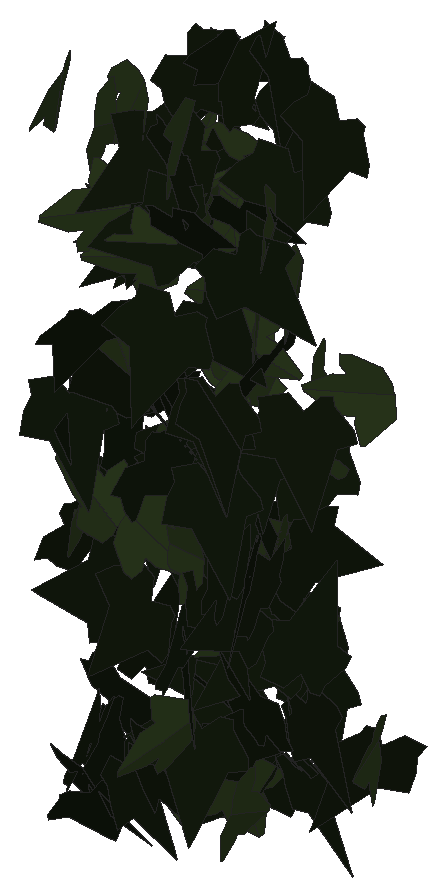
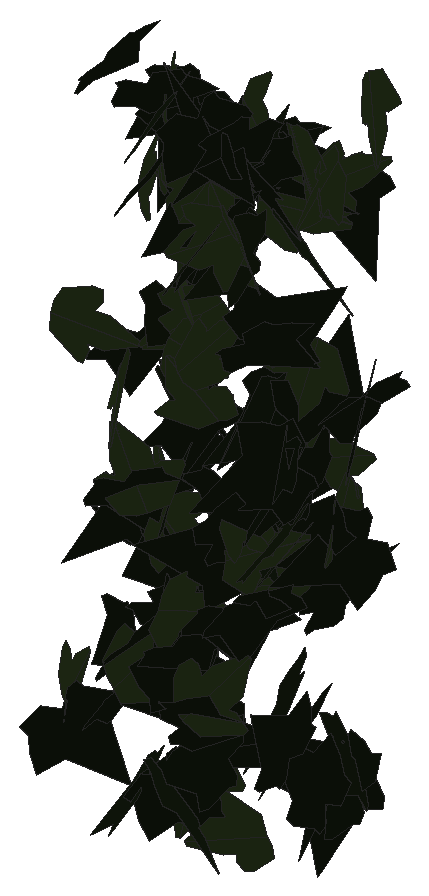
# SketchUp Ruby script. Lengths in inches.
U = 1.inch
M = Sketchup.active_model
def pt(a) = Geom::Point3d.new(a.map { |v| v * U })
def face(e, loops, mat)
  f = e.add_face(loops[0].map { |a| pt(a) })
  loops[1..].each { |l| e.add_face(l.map { |a| pt(a) }).erase! }
  f.material = f.back_material = mat if mat
  f
end
# faces: each face lists its corners as indices into pts; further lists are holes
def faces(e, pts, list, mat = nil) = list.each { |f| face(e, (f[0].is_a?(Array) ? f : [f]).map { |l| l.map { |i| pts[i] } }, mat) }
# xy, xz, yz: faces in a plane at the given z, y or x. An outline is a flat list of corners, or four numbers for a rectangle; further outlines are holes
def ring(l) = l.size == 4 ? [[l[0], l[1]], [l[2], l[1]], [l[2], l[3]], [l[0], l[3]]] : l.each_slice(2).to_a
def flat(e, list, mat, &to3) = list.each { |f| face(e, (f[0].is_a?(Array) ? f : [f]).map { |l| ring(l).map { |u, v| to3.(u, v) } }, mat) }
def xy(e, z, list, mat = nil) = flat(e, list, mat) { |x, y| [x, y, z] }
def xz(e, y, list, mat = nil) = flat(e, list, mat) { |x, z| [x, y, z] }
def yz(e, x, list, mat = nil) = flat(e, list, mat) { |y, z| [x, y, z] }
def lines(e, pts, list) = list.each { |a, b| e.add_line(pt(pts[a]), pt(pts[b])) }
# prism: a flat outline (further loops are holes) pulled along v
def prism(e, loops, v, mat = nil)
  f = face(e, loops, mat); d = Geom::Vector3d.new(v.map { |x| x * U })
  f.pushpull(f.normal.samedirection?(d) ? d.length : -d.length)
end
def box(e, o, s, mat = nil) = prism(e, [[o, [o[0] + s[0], o[1], o[2]], [o[0] + s[0], o[1] + s[1], o[2]], [o[0], o[1] + s[1], o[2]]]], [0, 0, s[2]], mat)
def at(x, y, z, deg = 0) = Geom::Transformation.translation(pt([x, y, z])) * Geom::Transformation.rotation(ORIGIN, Z_AXIS, deg.degrees)
def axes(o, x, y, z) = Geom::Transformation.new([*x, 0, *y, 0, *z, 0, *pt(o).to_a, 1])
def part(name) = M.definitions.add(name)
# library, detail: a bought-in or finely detailed component or shape, given as its bounding box
def library(name, o, s) = part(name).tap { |d| box(d.entities, o, s) }
def detail(e, o, s) = box(e.add_group.entities, o, s)
def put(e, d, t, mat = nil) = e.add_instance(d, t).tap { |i| i.material = mat if mat }
def group(e, t, mat = nil) = e.add_group.tap { |g| g.transformation = t; g.material = mat if mat }.entities
root = M.entities
M.materials.add("efeu1").color = [18, 25, 13]
M.materials.add("efeu2").color = [43, 57, 29]
c1 = part("ivyleaf_9")
p = [[1.54,2.16,1.25],[1.36,2.04,1.19],[-0.21,0.99,0.68],[-0.71,1.11,0.82],[-0.85,0.86,0.67],[-0.8,0.17,0.21],
  [-0.9,-0.01,0.1],[-0.67,-0.16,-0.02],[-0.08,-0.08,-0.05],[-0.03,-0.6,-0.4],[0.65,-0.88,-0.66],[0.83,-0.6,-0.49],
  [1.29,-0.42,-0.43],[1.8125,-0.07,-0.26],[1.21,0.44,0.15]]
faces(c1.entities,p,[[0,1,2,3,4,5,6,7,8,9,10,11,12,13,14]],"efeu1")
c2 = part("ivyleaf_10")
p = [[0,0.5,-0.03],[-0.0625,2.02,-0.43],[-0.19,2.01,-0.46],[-0.54,1.05,-0.29],[-0.52,0.625,-0.18],[-0.83,0.76,-0.28],
  [-1.16,0.64,-0.33],[-1.15,0.33,-0.24],[-0.77,-0.39,0.02],[-0.3,-0.51,0.16],[0.04,-0.48,0.23],[-0.02,2.01,-0.4375],
  [-0.06,2.01,-0.43],[0.04,-0.49,0.23],[0.67,-0.49,0.14],[1.38,0.36,-0.2],[1.375,0.51,-0.24],[0.81,0.65,-0.19],
  [0.62,0.59,-0.15],[0.6,1.09,-0.28],[0.5,1.23,-0.31]]
faces(c2.entities,p,[[0,1,2,3,4,5,6,7,8,9,10],[11,12,0,13,14,15,16,17,18,19,20]],"efeu2")
put(root,c1,axes([37.8,221.21,223.68],[0.09366,-0.09752,0.48137],[0.35058,-0.32993,-0.13506],[0.34398,0.36281,0.00657]))
put(root,c1,axes([38.375,219.91,223.58],[0.02364,0.24467,0.43541],[-0.069,0.43331,-0.23974],[-0.49465,-0.04875,0.05425]))
put(root,c2,axes([38.27,219.55,233.58],[0.1026,-0.46256,-0.15972],[-0.0382,0.15512,-0.47379],[0.48787,0.10943,-0.00351]))
put(root,c1,axes([38.21,221.43,224.3],[-0.06862,-0.15046,0.47186],[0.23997,0.40661,0.16456],[-0.43325,0.24905,0.01641]))
put(root,c1,axes([38.37,220.29,223.71],[0.09712,-0.08424,-0.48319],[-0.36952,0.31133,-0.12855],[0.32252,0.38207,-0.00178]))
put(root,c2,axes([38.31,220.36,232.64],[0.01185,-0.19518,-0.46018],[0.03052,0.45973,-0.19421],[0.49893,-0.02348,0.02281]))
put(root,c1,axes([38.17,219.9,226.92],[-0.0158,0.1862,-0.46376],[-0.03618,0.46235,0.18687],[0.49844,0.03946,-0.00114]))
put(root,c1,axes([38.4,222.04,230.77],[-0.32041,-0.35269,0.15149],[-0.10331,-0.11081,-0.4765],[0.36968,-0.33665,-0.00187]))
put(root,c1,axes([38.34,219.93,228.12],[-0.06556,0.01767,0.49537],[-0.03154,-0.49882,0.01362],[0.49468,-0.02946,0.06652]))
put(root,c1,axes([38.74,221.24,230.4],[0.08388,-0.01017,0.49281],[-0.4844,0.09082,0.08432],[-0.09123,-0.49158,0.00539]))
put(root,c2,axes([38.51,219.78,227.43],[0.06408,-0.33011,-0.37003],[0.00126,0.37322,-0.33273],[0.49588,0.04171,0.04866]))
put(root,c1,axes([38.6,220.32,225.93],[-0.105,-0.08425,0.48154],[-0.2914,-0.38467,-0.13084],[0.39251,-0.30812,0.03168]))
put(root,c1,axes([38.35,219.69,228.93],[0.02029,-0.48656,-0.11337],[0.01966,0.11415,-0.4864],[0.4992,0.01528,0.02376]))
put(root,c1,axes([38.58,220.46,227.85],[-0.04029,-0.15588,0.47337],[0.16236,0.4449,0.16033],[-0.47119,0.16663,0.01477]))
put(root,c1,axes([38.15,220.0625,223.17],[0.33116,-0.23651,0.29051],[0.24227,-0.16053,-0.40686],[0.28572,0.41024,0.00828]))
put(root,c2,axes([38.67,220.6,233.11],[0.38557,-0.25448,-0.19124],[-0.13642,0.13931,-0.46041],[0.28761,0.40723,0.038]))
put(root,c1,axes([38.66,219.77,223.23],[0.22546,0.44087,-0.06926],[-0.04183,-0.05638,-0.49505],[-0.44432,0.22903,0.01146]))
put(root,c1,axes([38.59,220.16,228.7],[0.37372,0.11242,0.31256],[-0.30078,-0.08507,0.39025],[0.14092,-0.47971,0.00404]))
put(root,c1,axes([38.6,221.04,228.71],[0.42532,-0.0676,-0.25404],[-0.25288,0.02676,-0.43051],[0.0718,0.49469,-0.01143]))
put(root,c1,axes([38.58,221.75,226.57],[-0.08422,-0.46567,-0.16143],[0.01454,0.16135,-0.47303],[0.49264,-0.08437,-0.01363]))
put(root,c1,axes([38.45,221.09,228.47],[0.40359,0.16044,0.24773],[0.21602,0.1254,-0.43314],[-0.20112,0.45666,0.0319]))
put(root,c1,axes([38.56,221.07,227.08],[0.0755,-0.45992,0.18102],[0.04637,-0.17572,-0.4658],[0.49209,0.08712,0.01612]))
put(root,c1,axes([38.6,221.46,227.22],[-0.03424,-0.39071,0.31011],[0.09378,-0.31034,-0.38065],[0.48993,0.0321,0.09453]))
put(root,c2,axes([39.12,219.48,227.64],[0.24319,0.08323,0.42887],[-0.43098,-0.03466,0.25111],[0.07152,-0.4918,0.05488]))
put(root,c2,axes([38.82,220.2,229.63],[-0.49191,-0.05886,-0.06754],[0.06744,0.00491,-0.49541],[0.05898,-0.4965,0.00311]))
put(root,c2,axes([38.98,221.47,227.13],[0.02043,0.03241,-0.49853],[-0.29026,-0.40532,-0.03824],[-0.40661,0.29097,0.00225]))
put(root,c1,axes([39.04,221.88,227.48],[-0.14516,-0.05957,0.47474],[-0.37338,-0.29612,-0.15132],[0.29919,-0.39845,0.04148]))
put(root,c1,axes([38.6,220.49,226.93],[-0.15026,-0.00193,0.47688],[0.47683,0.00755,0.15027],[-0.00778,0.49994,-0.00043]))
put(root,c1,axes([38.77,222,226.58],[-0.17085,-0.45556,-0.1152],[0.0422,0.10721,-0.48654],[0.468,-0.17598,0.00181]))
put(root,c2,axes([38.89,221.61,227.87],[-0.00604,-0.39503,0.30645],[0.05429,-0.30518,-0.39232],[0.49701,0.02853,0.04658]))
put(root,c2,axes([39,219.68,231.93],[-0.01634,0.10126,0.48937],[-0.08212,-0.48352,0.09731],[0.49294,-0.07719,0.03243]))
put(root,c2,axes([38.76,221.61,231.53],[0.41683,-0.2476,-0.12224],[0.11745,-0.04133,0.48425],[-0.24991,-0.43242,0.02371]))
put(root,c1,axes([39.23,220.17,231.45],[-0.4315,0.2526,0.00107],[-0.0024,-0.00198,-0.49999],[-0.25259,-0.4315,0.00292]))
put(root,c1,axes([38.86,221.43,231.72],[0.4296,-0.25429,0.02784],[0.02809,-0.00719,-0.49916],[0.25427,0.43044,0.0081]))
put(root,c1,axes([39.33,220.45,232.51],[-0.27676,-0.29301,0.29589],[-0.20834,-0.2102,-0.40301],[0.36056,-0.34636,-0.00574]))
put(root,c2,axes([38.87,221.37,222.83],[0.12734,0.07515,0.47764],[0.4279,0.21247,-0.14751],[-0.22514,0.44633,-0.01021]))
put(root,c1,axes([39.05,221.27,233.43],[0.16944,-0.24814,-0.39965],[-0.055,0.41142,-0.27877],[0.46719,0.13843,0.11213]))
put(root,c2,axes([39.5,221.75,224.75],[-0.35826,-0.09016,-0.33693],[-0.32121,-0.10293,0.36909],[-0.13592,0.48091,0.01583]))
put(root,c1,axes([39.67,221.43,223.95],[-0.37897,-0.04445,0.32312],[-0.31683,-0.06748,-0.38088],[0.07747,-0.49343,0.02298]))
put(root,c1,axes([39.71,221.75,224.35],[-0.29898,0.00793,0.40068],[-0.40032,-0.02949,-0.29812],[0.0189,-0.49907,0.02398]))
put(root,c1,axes([39.23,219.74,223.83],[0.27085,-0.32186,-0.27027],[-0.1674,0.21232,-0.42059],[0.38551,0.31832,0.00726]))
put(root,c2,axes([39.71,219.8,231.42],[-0.04376,-0.01549,0.49784],[-0.39942,-0.29748,-0.04437],[0.29757,-0.40158,0.01366]))
put(root,c1,axes([39.52,221.68,233.59],[-0.01844,0.29436,-0.40375],[0.04165,-0.40171,-0.29477],[-0.49792,-0.0445,-0.0097]))
put(root,c2,axes([39.15,221.68,231.98],[-0.28268,0.05148,-0.4092],[0.4033,-0.06927,-0.28732],[-0.08627,-0.49249,-0.00236]))
put(root,c1,axes([39.03,220.8,227.14],[0.24873,-0.22321,0.3719],[0.31582,-0.20066,-0.33165],[0.29731,0.39989,0.04116]))
put(root,c1,axes([39.61,220.71,232.51],[-0.48849,0.03449,-0.10093],[0.1011,-0.00113,-0.48967],[-0.03401,-0.49881,-0.00587]))
put(root,c1,axes([39.27,222.12,231.83],[0.07581,-0.4456,0.21377],[0.04073,-0.2099,-0.45198],[0.49254,0.08594,0.00447]))
put(root,c1,axes([39.33,221.3125,227.93],[-0.28695,-0.23006,-0.33872],[0.30487,0.15607,-0.36428],[0.27334,-0.41559,0.05071]))
put(root,c2,axes([39.54,221.74,229.97],[-0.0059,0.22333,0.44731],[0.01772,-0.44697,0.22339],[0.49965,0.01849,-0.00264]))
put(root,c1,axes([39.27,220.4,228.64],[0.45387,-0.20582,0.04051],[0.03764,-0.01507,-0.49835],[0.20636,0.45543,0.00181]))
put(root,c1,axes([39.18,221.58,223.99],[0.41756,-0.17367,0.21327],[0.19997,-0.0745,-0.45218],[0.18884,0.46291,0.00724]))
put(root,c1,axes([39.97,219.97,231.81],[-0.38802,0.01403,0.31503],[-0.31529,-0.00794,-0.38798],[-0.00589,-0.49974,0.01501]))
put(root,c1,axes([39.51,219.66,224.22],[0.36831,-0.18622,-0.28226],[-0.23213,0.16426,-0.41126],[0.2459,0.43398,0.03454]))
put(root,c1,axes([39.78,218.34,231.19],[0.00691,0.41592,-0.27741],[-0.0088,-0.2773,-0.41597],[-0.49987,0.01063,0.00349]))
put(root,c1,axes([39.47,221.43,232.96],[-0.2116,0.22995,0.39032],[0.26819,-0.28361,0.31247],[0.3651,0.3416,-0.00331]))
put(root,c1,axes([39.28,221.125,226.78],[0.28058,-0.00538,0.41382],[0.4137,-0.00986,-0.28063],[0.01118,0.49987,-0.00108]))
put(root,c1,axes([39.54,221.11,231.92],[0.1708,-0.37712,-0.28037],[-0.08251,0.26961,-0.41292],[0.46262,0.18732,0.02986]))
put(root,c1,axes([39.68,221.98,225.6875],[-0.2042,-0.45622,-0.01283],[0.00557,0.01156,-0.49984],[0.45637,-0.20428,0.00037]))
put(root,c1,axes([39.5,220.55,232.48],[0.05332,-0.37676,0.32436],[0.11545,-0.30792,-0.37664],[0.48356,0.11506,0.05416]))
put(root,c2,axes([39.68,220.38,233.16],[0.16846,-0.37973,0.27826],[0.16625,-0.22851,-0.41249],[0.44043,0.23149,0.04928]))
put(root,c1,axes([39.75,219.53,228.56],[0.00231,-0.03094,-0.49904],[-0.16684,0.47039,-0.02993],[0.47134,0.16666,-0.00815]))
put(root,c2,axes([39.91,221.79,226.12],[0.07806,0.18942,-0.4561],[-0.21368,-0.40335,-0.20409],[-0.44525,0.22678,0.01798]))
put(root,c2,axes([39.89,220.71,231.98],[0.07426,-0.49203,-0.04892],[-0.00776,0.0483,-0.4976],[0.49439,0.07466,-0.00046]))
put(root,c1,axes([40.11,221.64,223.41],[-0.34663,0.35961,0.02292],[-0.01635,0.01607,-0.49947],[-0.35997,-0.34702,0.00061]))
put(root,c2,axes([39.64,221.35,229.03],[0.4277,0.09238,-0.24194],[0.22365,0.10379,0.43498],[0.13059,-0.48031,0.04746]))
put(root,c2,axes([39.73,219.42,227.66],[0.1294,0.35556,0.32685],[0.07547,0.31933,-0.37727],[-0.47703,0.14698,0.02898]))
put(root,c1,axes([40.1,221.61,223.39],[-0.02246,0.14238,-0.47877],[-0.09415,-0.47187,-0.13591],[-0.49054,0.08405,0.04801]))
put(root,c1,axes([39.84,221.67,224.98],[0.20631,0.36397,0.27379],[-0.19506,-0.20099,0.41419],[0.41157,-0.27771,0.05905]))
put(root,c1,axes([39.95,219.29,226.68],[-0.13965,-0.37668,0.29767],[-0.10693,-0.27781,-0.40173],[0.46804,-0.17586,-0.00297]))
put(root,c2,axes([40.06,220.99,223.35],[-0.2418,-0.40591,-0.16362],[0.09503,0.13378,-0.47231],[0.4272,-0.25951,0.01246]))
put(root,c2,axes([40.48,219.48,227.49],[0.1014,-0.07931,-0.48314],[-0.3879,0.28805,-0.12869],[0.29875,0.40092,-0.00311]))
put(root,c1,axes([40.4,219.33,225.94],[-0.00066,0.26941,0.42121],[-0.10476,0.41179,-0.26355],[-0.4889,-0.0886,0.05591]))
put(root,c1,axes([39.96,220.75,231.83],[-0.07164,-0.11151,-0.48211],[0.26064,0.40558,-0.13254],[0.42063,-0.27031,0.00002]))
put(root,c2,axes([40.41,220.63,232.08],[0.4204,-0.18573,-0.19689],[-0.18495,0.06843,-0.45947],[0.19762,0.45915,-0.01117]))
put(root,c1,axes([40.12,222.08,232.73],[0.05267,-0.46125,0.18568],[0.01466,-0.18519,-0.46421],[0.497,0.05434,-0.00598]))
put(root,c1,axes([40.17,219.57,232.22],[0.47432,0.12821,-0.09262],[-0.08966,-0.02323,-0.49135],[-0.1303,0.48272,0.00096]))
put(root,c1,axes([40.11,221.95,233.46],[0.05779,-0.42634,0.25475],[0.03502,-0.25233,-0.43024],[0.49541,0.06757,0.0007]))
put(root,c2,axes([40.06,220.93,232.05],[0.39082,0.16969,0.26166],[0.24109,0.10172,-0.42606],[-0.19782,0.4592,-0.00231]))
put(root,c2,axes([40.37,220.96,229.5625],[-0.08436,-0.30374,0.3881],[0.01658,-0.39528,-0.30575],[0.49255,-0.03872,0.07676]))
put(root,c2,axes([40.45,222.09,225.0625],[-0.0941,-0.16956,-0.46086],[-0.21028,-0.41014,0.19383],[-0.44377,0.2303,0.00588]))
put(root,c2,axes([40.45,221.19,226.98],[-0.04781,-0.42423,0.26028],[-0.02472,-0.25913,-0.4269],[0.49709,-0.05369,0.00381]))
put(root,c1,axes([40.13,220.48,224.18],[0.10169,0.25804,-0.41602],[0.12304,0.39779,0.27681],[0.47383,-0.15868,0.0174]))
put(root,c1,axes([40.27,220.04,230.77],[0.15807,-0.28464,-0.37947],[-0.12656,0.36017,-0.32289],[0.45716,0.19813,0.04181]))
put(root,c2,axes([40.2,220.7,230.04],[-0.26791,-0.12344,-0.40372],[0.38427,0.1267,-0.29374],[0.17482,-0.46766,0.02699]))
put(root,c1,axes([40.33,220.83,228.4375],[-0.0896,-0.46721,-0.1539],[0.01753,0.1533,-0.4756],[0.49159,-0.09062,-0.01109]))
put(root,c2,axes([40.49,219.19,225.08],[0.01642,-0.12492,0.48387],[0.0185,-0.48364,-0.12549],[0.49939,0.02203,-0.01126]))
put(root,c1,axes([40.61,221.06,227.03],[0.03746,-0.35055,0.35456],[-0.01948,0.35426,0.35231],[-0.49821,-0.04021,0.01289]))
put(root,c2,axes([40.36,221.87,227.74],[-0.39971,-0.23086,0.19219],[0.18881,0.05572,0.45961],[-0.23363,0.44,0.04264]))
put(root,c1,axes([40.68,221.11,225.625],[-0.4175,-0.23326,0.14588],[-0.11975,-0.08462,-0.47802],[0.24769,-0.43408,0.0148]))
put(root,c1,axes([40.5,222,227.9],[-0.29139,-0.39579,-0.09186],[0.04993,0.0773,-0.49146],[0.40323,-0.29559,-0.00553]))
put(root,c1,axes([40.41,222.05,225.51],[-0.05188,-0.48145,0.12456],[-0.01912,-0.12321,-0.4842],[0.49693,-0.05501,-0.00563]))
put(root,c1,axes([40.27,219.62,225.83],[0.0335,-0.08517,-0.49155],[0.48386,-0.1144,0.0528],[-0.12146,-0.47923,0.07475]))
put(root,c1,axes([40.49,219.67,224.8],[-0.18841,-0.44969,-0.11082],[0.04089,0.10302,-0.48756],[0.46134,-0.19278,-0.00205]))
put(root,c2,axes([40.33,221.03,230.57],[0.1586,-0.1335,0.455],[0.34672,-0.29464,-0.20731],[0.32347,0.38127,-0.00089]))
put(root,c1,axes([40.83,220.62,230],[-0.20595,0.42196,-0.17184],[0.06691,-0.15853,-0.46946],[-0.45067,-0.21637,0.00883]))
put(root,c1,axes([40.33,221.27,226.52],[-0.0562,-0.09041,-0.48854],[0.46817,0.15495,-0.08253],[0.16632,-0.46671,0.06724]))
put(root,c1,axes([40.41,221.84,223.25],[0.31637,-0.38597,-0.03055],[-0.01653,0.02596,-0.49905],[0.38683,0.31678,0.00366]))
put(root,c2,axes([40.63,220.74,232.41],[-0.08905,-0.37665,0.31655],[0.17265,-0.32516,-0.33832],[0.46072,0.04905,0.18797]))
put(root,c1,axes([40.92,220.43,224.67],[0.2082,-0.22131,0.39709],[-0.27056,0.29065,0.30384],[-0.36531,-0.34139,0.00128]))
put(root,c1,axes([40.59,221.96,224.73],[0.09181,-0.4915,-0.00142],[0.00062,0.00156,-0.5],[0.4915,0.09181,0.0009]))
put(root,c2,axes([40.97,221.51,229.21],[-0.24738,0.25486,0.35192],[-0.24345,0.25413,-0.35517],[-0.35991,-0.34707,-0.00164]))
put(root,c2,axes([40.77,220.8125,226.8125],[0.14265,-0.44864,-0.16844],[0.07277,-0.15342,0.47028],[-0.47366,-0.15869,0.02152]))
put(root,c1,axes([40.6875,219.71,226.93],[0.21501,-0.45026,-0.03218],[-0.01225,0.02981,-0.49896],[0.45124,0.21535,0.00179]))
put(root,c1,axes([40.94,218.54,231.47],[-0.25571,-0.42954,0.01031],[-0.00532,-0.00884,-0.49989],[0.42963,-0.25577,-0.00005]))
put(root,c1,axes([41,219.89,232.5],[0.43121,0.18753,-0.16996],[-0.15838,-0.06196,-0.47019],[-0.19741,0.45934,0.00597]))
put(root,c1,axes([41.35,219.14,227.41],[-0.02938,0.18797,0.46239],[-0.20495,0.4178,-0.18286],[-0.45512,-0.20028,0.05249]))
put(root,c1,axes([41.01,220.96,227.1],[0.06007,0.04055,-0.49472],[-0.13137,0.48186,0.02355],[0.47868,0.12715,0.06854]))
put(root,c1,axes([40.97,219.33,228.74],[0.00134,-0.48087,-0.13696],[-0.00042,0.13696,-0.48087],[0.5,0.00141,-0.00004]))
put(root,c1,axes([41.04,219.29,230.01],[0.02647,-0.49465,-0.06799],[-0.01248,0.06741,-0.49528],[0.49914,0.02792,-0.00878]))
put(root,c1,axes([41.27,219.79,226.84],[-0.11284,-0.24663,0.42005],[-0.18799,-0.37571,-0.2711],[0.44936,-0.21911,-0.00794]))
put(root,c2,axes([41.31,219.37,224.08],[-0.01776,-0.236,-0.44044],[0.01288,0.44036,-0.23647],[0.49952,-0.01974,-0.00957]))
put(root,c1,axes([41.08,219.27,229.92],[0.09961,-0.48251,0.08522],[0.01435,-0.08405,-0.49268],[0.48977,0.1006,-0.0029]))
put(root,c1,axes([41.4,220.38,232.93],[-0.33829,-0.36508,-0.04774],[0.03004,0.03724,-0.49771],[0.36696,-0.33961,-0.00327]))
put(root,c1,axes([41.62,221.91,223.99],[-0.00766,0.22691,-0.44548],[-0.00447,-0.44555,-0.22687],[-0.49992,0.0005,0.00886]))
put(root,c1,axes([41.35,220.69,229.28],[-0.13585,-0.44094,-0.19265],[0.05225,0.18548,-0.46137],[0.47834,-0.14549,-0.00432]))
put(root,c1,axes([41.26,220.91,224.88],[-0.11095,-0.04659,-0.4853],[0.46751,0.13102,-0.11946],[0.1383,-0.48027,0.01449]))
put(root,c1,axes([41.875,219.15,227.375],[-0.07398,0.27785,0.40906],[-0.13769,0.38568,-0.28687],[-0.47494,-0.15509,0.01944]))
put(root,c2,axes([41.43,219.93,232.4],[-0.00917,0.02903,0.49907],[0.34846,-0.35754,0.0272],[0.35846,0.34831,-0.01368]))
put(root,c1,axes([41.66,220.27,225.89],[-0.41565,0.17428,0.21647],[0.20016,-0.08245,0.45071],[0.1928,0.46133,-0.00123]))
put(root,c2,axes([41.46,220.4,231.48],[0.04937,-0.17808,0.4646],[0.32269,-0.34392,-0.16611],[0.37873,0.31624,0.08097]))
put(root,c2,axes([42.03,221.28,229.58],[0.10555,-0.01546,-0.48849],[-0.48858,0.00894,-0.10585],[0.01201,0.49968,-0.01322]))
put(root,c1,axes([41.64,221.02,233.5],[-0.08641,-0.45584,0.18639],[-0.02449,-0.18503,-0.46386],[0.49187,-0.0893,0.00965]))
put(root,c1,axes([41.5,219.21,232.28],[-0.05239,-0.13832,-0.47762],[0.29929,0.37476,-0.14135],[0.39709,-0.30071,0.04353]))
put(root,c1,axes([41.73,219.21,228.03],[-0.19556,0.09664,-0.44991],[0.39795,-0.20996,-0.21807],[-0.23107,-0.44337,0.00521]))
put(root,c2,axes([41.76,221.69,224.15],[-0.01641,-0.02653,-0.49903],[0.07836,-0.49326,0.02365],[-0.49355,-0.07743,0.02034]))
